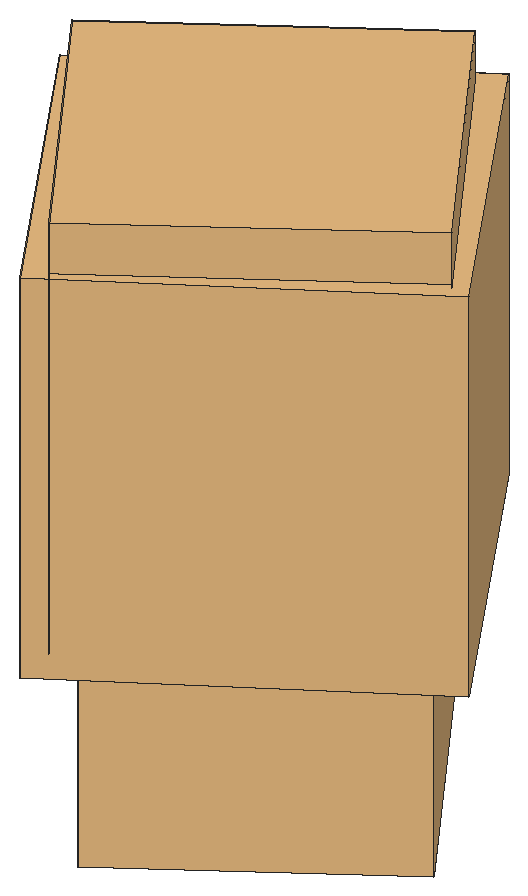
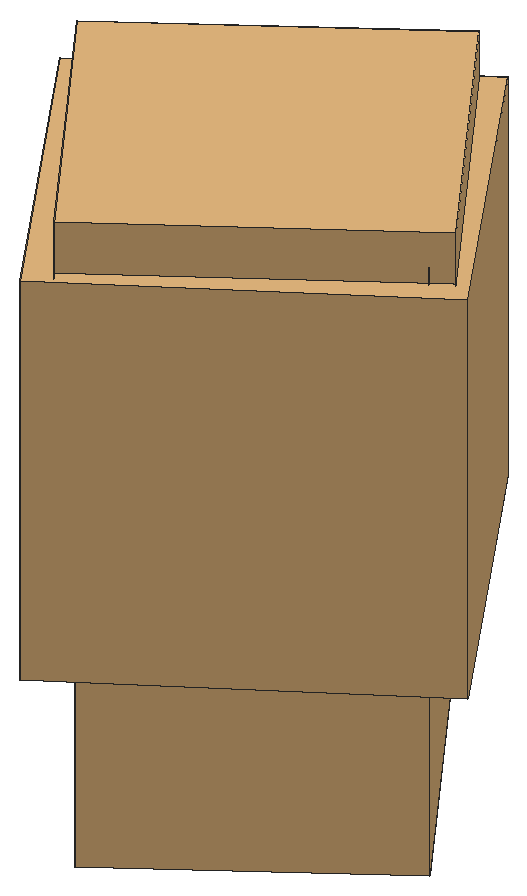
# SketchUp Ruby script. Lengths in inches.
U = 1.inch
M = Sketchup.active_model
def pt(a) = Geom::Point3d.new(a.map { |v| v * U })
def face(e, loops, mat)
  f = e.add_face(loops[0].map { |a| pt(a) })
  loops[1..].each { |l| e.add_face(l.map { |a| pt(a) }).erase! }
  f.material = f.back_material = mat if mat
  f
end
# faces: each face lists its corners as indices into pts; further lists are holes
def faces(e, pts, list, mat = nil) = list.each { |f| face(e, (f[0].is_a?(Array) ? f : [f]).map { |l| l.map { |i| pts[i] } }, mat) }
# xy, xz, yz: faces in a plane at the given z, y or x. An outline is a flat list of corners, or four numbers for a rectangle; further outlines are holes
def ring(l) = l.size == 4 ? [[l[0], l[1]], [l[2], l[1]], [l[2], l[3]], [l[0], l[3]]] : l.each_slice(2).to_a
def flat(e, list, mat, &to3) = list.each { |f| face(e, (f[0].is_a?(Array) ? f : [f]).map { |l| ring(l).map { |u, v| to3.(u, v) } }, mat) }
def xy(e, z, list, mat = nil) = flat(e, list, mat) { |x, y| [x, y, z] }
def xz(e, y, list, mat = nil) = flat(e, list, mat) { |x, z| [x, y, z] }
def yz(e, x, list, mat = nil) = flat(e, list, mat) { |y, z| [x, y, z] }
def lines(e, pts, list) = list.each { |a, b| e.add_line(pt(pts[a]), pt(pts[b])) }
# prism: a flat outline (further loops are holes) pulled along v
def prism(e, loops, v, mat = nil)
  f = face(e, loops, mat); d = Geom::Vector3d.new(v.map { |x| x * U })
  f.pushpull(f.normal.samedirection?(d) ? d.length : -d.length)
end
def box(e, o, s, mat = nil) = prism(e, [[o, [o[0] + s[0], o[1], o[2]], [o[0] + s[0], o[1] + s[1], o[2]], [o[0], o[1] + s[1], o[2]]]], [0, 0, s[2]], mat)
def at(x, y, z, deg = 0) = Geom::Transformation.translation(pt([x, y, z])) * Geom::Transformation.rotation(ORIGIN, Z_AXIS, deg.degrees)
def axes(o, x, y, z) = Geom::Transformation.new([*x, 0, *y, 0, *z, 0, *pt(o).to_a, 1])
def part(name) = M.definitions.add(name)
# library, detail: a bought-in or finely detailed component or shape, given as its bounding box
def library(name, o, s) = part(name).tap { |d| box(d.entities, o, s) }
def detail(e, o, s) = box(e.add_group.entities, o, s)
def put(e, d, t, mat = nil) = e.add_instance(d, t).tap { |i| i.material = mat if mat }
def group(e, t, mat = nil) = e.add_group.tap { |g| g.transformation = t; g.material = mat if mat }.entities
root = M.entities
M.materials.add("028_190k_fullGeometry_Material \#4").color = [120, 148, 64]
M.materials.add("0ad16as01f6asdLeafVar1sfd015as60f1as6").color = [231, 235, 211]
M.materials.add("asdfasdf0165f6asdLeafVar1sfd015as60f1as6").color = [231, 235, 211]
M.materials.add("dw_stemssadfasdfa0sdf1s01d6w1").color = [90, 97, 50]
M.materials.add("viburnumblaasdfas0df1w06d").color = [98, 102, 84]
M.materials.add("viburnumbladsadfasdfad0w122").color = [125, 129, 119]
c1 = part("Component\#314")
p = [[0.14,0,0],[2.58,0.05,0.25],[2.44,5.11,2.64],[0,5.05,2.39]]
faces(c1.entities,p,[[0,1,2,3]],"viburnumblaasdfas0df1w06d")
c2 = part("viburnumblad1\#2")
put(c2.entities,c1,axes([-37.25,6.23,19.31],[75.98784,0,0],[0,65.50676,0],[0,0,75.98784]))
c3 = library("028_190k_fullGeometry_0",[-319.99,-281.1,-2.15],[577.33,562.38,1159.36])
c4 = library("028_190k_fullGeometry_1",[-333.4,-281.7,421.48],[600.33,578.53,738.83])
c5 = library("028_190k_fullGeometry_2",[-3584003,-3264710,4041818.25],[6566285.5,6460741.75,7903602.75])
c6 = library("028_190k_fullGeometry_3",[-353.86,-324.57,405.22],[652.24,636.69,781.83])
c7 = part("028_190k_fullGeometry_4")
p = [[125.51,152.8,882.93],[125.36,152.82,883.01],[124.8,155.5625,881.05]]
faces(c7.entities,p,[[0,1,2]],"028_190k_fullGeometry_Material \#4")
c8 = part("028_190k_fullGeometry")
g1 = group(c8.entities,at(0,0,0))
put(g1,c3,axes([0,0,0],[0.18998,-0.26642,0],[0.26642,0.18998,0],[0,0,0.32722]))
put(g1,c4,axes([0,0,0],[0.18998,-0.26642,0],[0.26642,0.18998,0],[0,0,0.32722]))
put(g1,c5,axes([0,0,0],[0.00002,-0.00003,0],[0.00003,0.00002,0],[0,0,0.00003]))
put(g1,c6,axes([0,0,0],[0.18998,-0.26642,0],[0.26642,0.18998,0],[0,0,0.32722]))
put(g1,c7,axes([0,0,0],[0.18998,-0.26642,0],[0.26642,0.18998,0],[0,0,0.32722]))
c9 = part("Component\#315")
p = [[0.25,0,0],[2.05,0.01,0.35],[1.81,4.2,1.66],[0,4.19,1.3125]]
faces(c9.entities,p,[[0,1,2,3]],"viburnumbladsadfasdfad0w122")
c10 = part("viburnumblad2")
put(c10.entities,c9,axes([-19.23,-4.49,-32.18],[83.35428,0,0],[0,79.38502,0],[0,0,83.35428]))
c11 = part("vdw_leaf\#1")
p = [[0,0,0],[-2.77,1.61,2.32],[-4.3125,6.1,4.5],[-3.97,13.49,6.09],[-2.47,18.57,6.3],[-0.2,22.73,5.75],
  [2.54,19.66,6.85],[4.3,15.93,7.09],[5.03,7.6,5.43],[3.32,1.76,2.74]]
faces(c11.entities,p,[[0,1,2,3,4,5],[0,5,6,7,8,9]],"0ad16as01f6asdLeafVar1sfd015as60f1as6")
c12 = part("dw_branch_3\#2")
p = [[-10.06,-1.6,62.9],[-0.2,1.54,-0.01],[-10.43,1.54,62.72],[0.18,-1.6,0.17],[-23.75,-21.66,88.91],[-25.7,-20.3,89.55],
  [13.4,11.62,104.56],[13.33,13.52,104.47],[-49.25,-41.87,130.3125],[-50.33,-40.21,130.71],[-4.97,21.13,143.98],[35.61,27.99,178.64],
  [-5.09,23.64,143.96],[35.32,29.14,178.46],[-67.7,-55.38,181.06],[-68.34,-54.45,181.62],[-22.8125,33.9,200.59],[-22.94,35.79,200.41],
  [56.61,36.78,229.75],[56.29,38.09,229.57],[-70.63,-67.46,248.85],[-70.72,-66.33,249.5],[-25.05,43.32,240.75],[-24.98,44.26,240.57]]
faces(c12.entities,p,[[0,1,2],[0,3,1],[4,2,5],[4,0,2],[6,0,2],[6,2,7],[8,4,5],[8,5,9],
  [10,6,7],[11,6,7],[10,7,12],[11,7,13],[14,8,9],[14,9,15],[16,10,12],[16,12,17],
  [18,11,13],[18,13,19],[20,14,15],[20,15,21],[22,16,17],[22,17,23]],"dw_stemssadfasdfa0sdf1s01d6w1")
c13 = part("dw_branch3\#2")
put(c13.entities,c11,axes([-70.33,-63.58,233.32],[-1.00752,0.412,0.78596],[-0.24851,-1.22189,0.32195],[0.83141,0.09817,1.01433]))
put(c13.entities,c11,axes([-66.93,-54.91,182.82],[-0.84976,-0.98359,0.33619],[0.99572,-0.74889,0.32577],[-0.05223,0.46521,1.22907]))
put(c13.entities,c11,axes([-46.12,-39.49,126.35],[1.23843,0.5364,0.23552],[-0.56438,0.94474,0.81599],[0.15707,-0.83465,1.07498]))
put(c13.entities,c11,axes([13.0625,13.13,104.77],[-1.01271,0.69982,-0.26884],[-0.74268,-0.99813,0.19939],[-0.10222,0.31872,1.21473]))
put(c13.entities,c11,axes([-18.87,30.42,186.42],[0.36309,1.06515,-0.56675],[-1.14134,0.49515,0.19939],[0.39128,0.45593,1.10754]))
put(c13.entities,c11,axes([-3.2,4.15,75.77],[-1.04153,0.55414,0.44243],[-0.23365,-1.01045,0.71554],[0.6695,0.50943,0.93801]))
put(c13.entities,c11,axes([23.2,19.41,136.3],[-0.65687,-1.11295,-0.05714],[1.05857,-0.61429,-0.20411],[0.15163,-0.1536,1.24868]))
put(c13.entities,c11,axes([-25.57,35.48,201.32],[-0.64726,0.62827,0.87973],[-0.71635,-1.0172,0.19939],[0.80962,-0.39773,0.87973]))
put(c13.entities,c11,axes([-36.37,-32.14,110.35],[-0.80747,1.09962,0.12544],[-0.83333,-0.50188,-0.96467],[-0.72833,-0.64487,0.96467]))
put(c13.entities,c11,axes([-9.89,26.72,156.79],[0.45529,1.02969,0.56572],[-1.16919,0.33753,0.32662],[0.11537,-0.64297,1.07744]))
put(c13.entities,c11,axes([-26.57,46.1,241.0625],[0.00015,0.80921,0.22536],[-0.83985,0.00446,-0.01542],[-0.01605,-0.22532,0.80906]))
put(c13.entities,c11,axes([-9.2,-2.58,61.06],[-1.10001,-0.40312,0.39014],[0.40883,-1.1116,0.00411],[0.35732,0.13566,1.14763]))
put(c13.entities,c11,axes([-69.91,-63.11,233.93],[1.36249,-0.1432,0],[0.13201,1.25603,0.5309],[-0.05549,-0.52799,1.26295]))
put(c13.entities,c11,axes([32.2,25.46,166.13],[0.06878,-1.29051,-0.05714],[1.22165,0.07415,-0.20411],[0.2113,-0.04403,1.24868]))
put(c13.entities,c11,axes([-5.68,-0.66,44.43],[-0.48448,-1.12287,0.17078],[0.98138,-0.33653,0.57135],[-0.48308,0.36756,1.04626]))
put(c13.entities,c11,axes([43.45,32.81,198.64],[0.5408,1.19584,0.14106],[-0.94242,0.32409,0.86557],[0.74952,-0.45533,0.98656]))
put(c13.entities,c11,axes([12.52,14.14,104.98],[1.02694,0.54888,0.41092],[-0.53566,1.05407,-0.06927],[-0.38969,-0.12321,1.13846]))
put(c13.entities,c11,axes([44.55,32.375,198.73],[-0.65687,-1.11295,-0.05714],[1.05857,-0.61429,-0.20411],[0.15163,-0.1536,1.24868]))
put(c13.entities,c11,axes([-5.67,21.17,141.44],[-1.10726,0.43603,-0.32953],[-0.49537,-1.03435,0.29588],[-0.17521,0.40597,1.12589]))
put(c13.entities,c11,axes([55.69,37.84,229.48],[0.18984,0.96334,0.18958],[-0.71996,0.0053,0.69399],[0.66755,-0.26823,0.69457]))
put(c13.entities,c11,axes([-21.52,36.85,205.2],[0.72606,-0.98817,0.14519],[0.94364,0.7084,0.10251],[-0.16885,0.05176,1.19664]))
put(c13.entities,c11,axes([-68.51,-56.35,196.07],[1.16319,0.72381,0],[-0.66725,1.0723,0.5309],[0.28049,-0.45075,1.26295]))
put(c13.entities,c12,at(0.01,-0.09,-0.02),"dw_stemssadfasdfa0sdf1s01d6w1")
put(c13.entities,c11,axes([-2.49,5.18,75.91],[0.78614,-0.90346,-0.30078],[0.86953,0.79562,-0.11715],[0.28546,-0.14014,1.16705]))
put(c13.entities,c11,axes([-23.125,-16.22,82.25],[0.32175,1.32576,0.12544],[-1.33153,0.31835,0.05068],[0.01989,-0.13382,1.3633]))
put(c13.entities,c11,axes([-23.75,41.99,230.3],[0.85958,-0.87451,0.14519],[0.66531,0.75721,0.62192],[-0.54076,-0.36226,1.01955]))
put(c13.entities,c11,axes([27.07,22.48,149.34],[0.92952,-0.64745,-0.62467],[0.50188,1.074,-0.36637],[0.71693,0.02135,1.04468]))
put(c13.entities,c11,axes([17.66,16.25,119.93],[-0.91649,0.83891,-0.3601],[-0.87434,-0.77966,0.40896],[0.0492,0.54447,1.14321]))
put(c13.entities,c11,axes([-68.37,-54.54,181.63],[0.32047,1.28399,0.35434],[-1.33153,0.31835,0.05068],[-0.03484,-0.35624,1.32241]))
put(c13.entities,c11,axes([-28.98,-27.1,96.48],[-0.8814,-0.35966,-0.98523],[0.75246,-1.11336,-0.26672],[-0.73065,-0.71272,0.91382]))
put(c13.entities,c11,axes([-15.23,28.43,172.72],[-1.21149,0.11898,0.32517],[-0.09739,-1.25259,0.09551],[0.33228,0.0667,1.21356]))
put(c13.entities,c11,axes([-17.5625,31.23,186.85],[-0.49275,-1.12287,0.14519],[0.95014,-0.33653,0.62192],[-0.53717,0.36756,1.01955]))
put(c13.entities,c11,axes([26.7,21.22,149.39],[-1.00104,0.22334,0.83093],[0.36894,-1.0402,0.72406],[0.77731,0.78134,0.72643]))
put(c13.entities,c11,axes([-31.125,-24.87,97.38],[0.75482,-0.86936,0.69068],[-0.00159,0.80023,1.00899],[-1.08766,-0.58016,0.45842]))
put(c13.entities,c11,axes([-71.21,-66.73,248.67],[0.25207,0.96771,0],[-0.8921,0.23237,0.38752],[0.375,-0.09768,0.92186]))
put(c13.entities,c11,axes([-24.11,41.05,229.55],[-1.11612,0.51924,-0.26884],[-0.56394,-1.10897,0.19939],[-0.15444,0.29694,1.21473]))
put(c13.entities,c11,axes([6.75,8.37,91.63],[-0.33418,-1.12287,0.39014],[1.13558,-0.33653,0.00411],[0.10478,0.36756,1.14763]))
put(c13.entities,c11,axes([-26,45.89,241.63],[-0.26986,-0.70824,-0.32129],[0.56818,-0.39091,0.38449],[-0.49365,-0.09775,0.63011]))
put(c13.entities,c11,axes([3.74,17.32,124.35],[0.22441,1.22913,-0.16274],[-1.07812,0.11178,-0.64246],[-0.61228,0.25367,1.07162]))
put(c13.entities,c11,axes([-5.44,22.27,140.88],[1.2203,0.00475,0.31374],[-0.097,1.20386,0.35905],[-0.29841,-0.37189,1.1663]))
put(c13.entities,c11,axes([-13.79,29.35,173.31],[0.83169,-0.90108,0.14519],[0.68877,0.73594,0.62192],[-0.55187,-0.34509,1.01955]))
put(c13.entities,c11,axes([-16.92,-7.26,72.98],[1.30647,0.30378,-0.27886],[0.07026,0.74892,1.14503],[0.40633,-1.10623,0.69861]))
put(c13.entities,c11,axes([4.8,17.55,125.22],[-0.25598,-1.17842,0.26559],[1.01553,-0.08455,0.60363],[-0.56975,0.35087,1.00767]))
put(c13.entities,c11,axes([5.3125,8.35,91.45],[0.00638,1.22913,-0.27714],[-1.16413,0.11178,0.46895],[0.48205,0.25367,1.13617]))
put(c13.entities,c11,axes([38.12,30.57,183.07],[1.12534,0.26182,-0.63833],[-0.46674,1.18829,-0.33545],[0.5081,0.51169,1.10563]))
put(c13.entities,c11,axes([-70.41,-60.38,214.47],[-0.41425,1.30587,0],[-1.20383,-0.38188,0.5309],[0.50605,0.16053,1.26295]))
put(c13.entities,c11,axes([37.03,28.75,180.67],[-1.12533,0.00102,-0.63799],[-0.00113,-1.2408,0],[-0.62497,0.00057,1.10237]))
put(c13.entities,c11,axes([30.71,25.35,165.96],[-0.1364,1.29314,0.22715],[-1.08768,-0.23921,0.70862],[0.73536,-0.11394,1.09026]))
put(c13.entities,c11,axes([-38.05,-30.84,110.67],[-0.31533,-1.27379,-0.2839],[1.018,-0.40311,0.67794],[-0.74394,-0.05723,1.08307]))
put(c13.entities,c11,axes([50.11,34.45,213.36],[-1.05669,0.74401,-0.05714],[-0.616,-0.82138,0.69675],[0.37221,0.60904,1.04705]))
put(c13.entities,c11,axes([-65.32,-58.78,200.07],[-1.14597,-0.19668,-0.6713],[0.21784,-1.26924,0],[-0.64812,-0.11124,1.139]))
put(c13.entities,c11,axes([-53.2,-43.37,143.59],[-0.72817,-1.09167,-0.2839],[0.82127,-0.72411,0.67794],[-0.71934,0.19815,1.08307]))
put(c13.entities,c11,axes([-61.1,-50.25,163.67],[-0.52887,1.19686,-0.30066],[-1.10762,-0.57104,-0.32484],[-0.42634,0.12264,1.23812]))
put(c13.entities,c11,axes([-54.12,-42.96,142.67],[0.32175,1.32576,0.12544],[-1.33153,0.31835,0.05068],[0.01989,-0.13382,1.3633]))
put(c13.entities,c11,axes([22.03,20.08,132.3],[1.17066,0.5058,-0.34078],[-0.35758,1.16671,0.50333],[0.49407,-0.35407,1.17172]))
put(c13.entities,c11,axes([-8.59,26.04,158.21],[-0.49275,-1.12287,0.14519],[0.95014,-0.33653,0.62192],[-0.53717,0.36756,1.01955]))
put(c13.entities,c11,axes([49.92,34.03,213.7],[1.24742,-0.35176,0.25024],[0.42127,1.159,-0.4708],[-0.09426,0.52477,1.20753]))
put(c13.entities,c11,axes([-70.34,-67.02,249.05],[-0.57048,-0.79684,0],[0.73827,-0.52855,0.24329],[-0.20203,0.14464,0.92729]))
put(c13.entities,c11,axes([56.04,36.81,228.63],[0.33451,-0.90845,-0.15237],[0.87636,0.33365,-0.06538],[0.11487,-0.11636,0.94597]))
put(c13.entities,c11,axes([-69.93,-60.58,214.88],[-0.45293,-0.99272,-0.78227],[1.14635,-0.58199,0.07483],[-0.40282,-0.65636,1.06615]))
put(c13.entities,c11,axes([-16.77,-8.59,72.7],[-1.22785,0.11509,0.53076],[-0.24879,-1.22495,-0.30991],[0.46742,-0.38989,1.16587]))
put(c13.entities,c11,axes([18.29,17.18,119.24],[1.19981,-0.45946,0.3029],[0.40159,1.22775,0.27158],[-0.37626,-0.1547,1.25575]))
put(c13.entities,c11,axes([-6.73,-0.68,43.74],[0.05346,1.22913,-0.27201],[-1.22696,0.11178,0.26396],[0.28163,0.25367,1.20164]))
put(c13.entities,c11,axes([-58.57,-48.42,160.98],[0.43385,-1.23789,0.39533],[1.04879,0.57965,0.66404],[-0.76727,0.09236,1.13122]))
put(c13.entities,c11,axes([-23.4,38.49,215.38],[0.06762,1.22913,-0.26884],[-1.23909,0.11178,0.19939],[0.21835,0.25367,1.21473]))
put(c13.entities,c11,axes([-22.21,-16.62,83.17],[-0.72817,-1.09167,-0.2839],[0.82127,-0.72411,0.67794],[-0.71934,0.19815,1.08307]))
put(c13.entities,c11,axes([-45.7,-40.77,126.53],[-1.33715,-0.0713,-0.0976],[0.07167,-1.28508,-0.04314],[-0.09306,-0.0492,1.31098]))
put(c13.entities,c11,axes([-22.39,38.51,216.12],[-0.49275,-1.12287,0.14519],[0.95014,-0.33653,0.62192],[-0.53717,0.36756,1.01955]))
c14 = part("vdw_leaf\#2")
p = [[0,0,0],[-2.77,1.61,2.32],[-4.3125,6.1,4.5],[-3.97,13.49,6.09],[-2.47,18.57,6.3],[-0.2,22.73,5.75],
  [2.54,19.66,6.85],[4.3,15.93,7.09],[5.03,7.6,5.43],[3.32,1.76,2.74]]
faces(c14.entities,p,[[0,1,2,3,4,5],[0,5,6,7,8,9]],"asdfasdf0165f6asdLeafVar1sfd015as60f1as6")
c15 = part("dg_branch_1\#2")
p = [[46.12,1.57,35.62],[46,5.42,35.41],[0.14,1.79,0.05],[0.26,-2.0625,0.27],[74.05,2.99,75.8],[74.11,5.28,75.58],
  [103.46,0.47,94.74],[104.03,2.92,94.84],[81.14,16.92,120.46],[81.2,18.78,120.24],[130.47,-5.6875,130.27],[130.58,-3.66,129.85],
  [80.82,34.4375,191.22],[80.64,35.93,190.9],[148.49,-14.56,203.24],[148.9,-12.8125,203.11],[81.08,37.95,226.93],[81.4,39.1,227.03],
  [157.45,-18.19,250.77],[157.7,-17.01,250.41]]
faces(c15.entities,p,[[0,1,2,3],[4,0,1],[4,1,5],[6,4,5],[6,5,7],[8,4,5],[8,5,9],[10,6,7],
  [10,7,11],[12,8,9],[12,9,13],[14,10,11],[14,11,15],[16,12,13],[16,13,17],[18,14,15],
  [18,15,19]],"dw_stemssadfasdfa0sdf1s01d6w1")
c16 = part("vdw_branch1\#3")
put(c16.entities,c14,axes([120.69,-2.42,117.31],[1.12221,-0.24063,-0.65809],[0.19207,1.24776,-0.12871],[0.65778,0.01392,1.11658]))
put(c16.entities,c14,axes([81,38.9,226.05],[0.7888,-0.58155,0],[0.48308,0.65523,0.47],[-0.28484,-0.38635,0.83138]))
put(c16.entities,c14,axes([78.08,12.69,106.05],[-1.43826,-0.02353,-0.03177],[0.0088,-1.31777,0.57755],[-0.03854,0.57714,1.31741]))
put(c16.entities,c14,axes([130.18,-4.73,130.41],[-0.38031,-1.29044,-0.11242],[1.20662,-0.31032,-0.51987],[0.47109,-0.24694,1.24081]))
put(c16.entities,c14,axes([157.08,-17.89,249.93],[-0.91355,0.40674,0],[-0.37496,-0.84216,0.38752],[0.15762,0.35401,0.92186]))
put(c16.entities,c14,axes([90.64,3.03,86.49],[0.32514,-0.85045,-0.99675],[0.69523,0.98247,-0.61148],[1.11061,-0.36604,0.67459]))
put(c16.entities,c14,axes([80.15,28.42,160.95],[-0.16039,0.95636,-1.06292],[-1.41646,0.03966,0.24943],[0.19509,1.07422,0.93709]))
put(c16.entities,c14,axes([126.74,-5.45,129.22],[-0.59819,0.96152,-0.6841],[-0.85772,0.12575,0.92675],[0.75427,0.88089,0.57856]))
put(c16.entities,c14,axes([133.22,-6.12,150.66],[-0.93823,0.76985,0.59124],[-0.47726,-1.08188,0.65135],[0.84525,0.24366,1.02405]))
put(c16.entities,c14,axes([80.43,22.89,141.32],[-1.42571,-0.19312,0.01373],[0.18338,-1.31425,0.5561],[-0.0621,0.5528,1.32692]))
put(c16.entities,c14,axes([33.14,0.88,26.42],[-0.13338,1.31536,0.04876],[-1.04528,-0.13221,0.7073],[0.72315,0.03348,1.07497]))
put(c16.entities,c14,axes([152.63,-15.08,221.76],[-1.28188,0.41945,0.0579],[-0.3638,-1.18547,0.53367],[0.21665,0.49113,1.23869]))
put(c16.entities,c14,axes([80.05,28.28,160.33],[-0.46732,-1.26661,0.40679],[1.27397,-0.40257,0.21004],[-0.07408,0.44645,1.30501]))
put(c16.entities,c14,axes([153.95,-14.8,235.875],[0.39005,1.07743,0.20605],[-0.96443,0.25296,0.50293],[0.42961,-0.3464,0.99807]))
put(c16.entities,c14,axes([80.2,24.22,141.74],[1.33062,-0.46576,0.02628],[0.44746,1.2746,-0.06608],[-0.00197,0.0722,1.37936]))
put(c16.entities,c14,axes([145.48,-12.5,188.92],[-1.32952,0.16983,0.16138],[-0.09299,-1.2361,0.53471],[0.21503,0.51548,1.22904]))
put(c16.entities,c14,axes([139.64,-9.18,171.24],[0.05682,1.30088,0.23414],[-1.13176,-0.05343,0.57151],[0.58357,-0.22963,1.13417]))
put(c16.entities,c14,axes([70.95,4.35,71.98],[-1.1081,-0.41873,0.64752],[0.33675,-1.28259,-0.25313],[0.6937,-0.04625,1.15721]))
put(c16.entities,c14,axes([59.85,4.55,56.17],[-0.26797,1.24526,0.35754],[-0.9369,-0.41634,0.74783],[0.83377,-0.10389,0.98674]))
put(c16.entities,c14,axes([33.11,3.36,25.66],[-0.57817,-1.07968,-0.5679],[1.11554,-0.21356,-0.7297],[0.49375,-0.78178,0.98363]))
put(c16.entities,c15,at(-0.21,0.34,-0.17),"dw_stemssadfasdfa0sdf1s01d6w1")
put(c16.entities,c14,axes([80.91,19.01,122.53],[-0.84258,1.13222,-0.27981],[-1.15093,-0.75138,0.42537],[0.18861,0.47293,1.3457]))
put(c16.entities,c14,axes([119.8,-1.22,114.1],[-1.3235,-0.25012,0.09101],[0.25933,-1.31572,0.15537],[0.05991,0.1698,1.33794]))
put(c16.entities,c14,axes([46.29,5.1,38.04],[0.98937,0.73827,-0.47585],[-0.72359,1.03721,0.10473],[0.44068,0.18581,1.20453]))
put(c16.entities,c14,axes([81.1875,33.03,184.45],[1.33883,0.26986,0.35053],[-0.09581,1.22087,-0.57399],[-0.42216,0.53228,1.20262]))
put(c16.entities,c14,axes([80.16,36.28,206.98],[-0.83993,0.85737,-0.6234],[-1.05964,-0.65701,0.5241],[0.02941,0.81391,1.07976]))
put(c16.entities,c14,axes([154.86,-16.15,234.87],[0.02509,-1.15302,-0.28506],[1.1487,-0.04894,0.29908],[-0.30202,-0.28195,1.11384]))
put(c16.entities,c14,axes([108.77,-0.33,101.14],[-0.47691,-1.03266,-0.72709],[1.25395,-0.29455,-0.40416],[0.15052,-0.81814,1.06325]))
put(c16.entities,c14,axes([89.79,3.01,85.87],[-0.61344,0.75518,0.8965],[-0.17758,-1.01824,0.73622],[1.13385,0.22574,0.58569]))
put(c16.entities,c14,axes([81.56,20.31,123.29],[0.37259,-1.3435,0.21057],[1.29385,0.32364,-0.22445],[0.16906,0.25791,1.34638]))
put(c16.entities,c14,axes([46.45,1.82,36.74],[-0.77883,0.29892,1.0614],[0.19124,-1.24314,0.49044],[1.08598,0.43329,0.67484]))
put(c16.entities,c14,axes([71.37,4.02,72.32],[0.72905,0.81546,-0.74421],[-0.66805,0.98958,0.42988],[0.8391,0.14186,0.97745]))
put(c16.entities,c14,axes([136.59,-5.88,150.53],[0.85845,-0.99897,-0.12437],[0.96526,0.81273,0.13453],[-0.02572,-0.18182,1.28292]))
put(c16.entities,c14,axes([80.375,38.8,225.86],[-0.25178,0.96778,0],[-0.89216,-0.23211,0.38752],[0.37503,0.09757,0.92186]))
put(c16.entities,c14,axes([74.43,7.99,85.38],[-1.05703,0.91669,-0.33543],[-0.95806,-0.87958,0.61531],[0.18697,0.6754,1.25659]))
put(c16.entities,c14,axes([76.57,9.74,89.32],[0.63146,-1.21538,0.33508],[1.18148,0.49387,-0.43517],[0.26321,0.48577,1.26593]))
put(c16.entities,c14,axes([81.6875,36.97,207.4],[0.09422,-1.04424,0.38486],[1.01646,0.1939,0.27727],[-0.33299,0.33382,0.98727]))
put(c16.entities,c14,axes([157.29,-17.17,249.98],[0.50586,-0.50586,0],[0.38853,0.38853,0.41105],[-0.29684,-0.29684,0.56115]))
put(c16.entities,c14,axes([79.92,15.8,106.09],[1.03917,-0.29343,-0.90675],[-0.14587,1.22131,-0.5624],[0.92163,0.5191,0.88824]))
put(c16.entities,c14,axes([61.95,3.88,56.26],[0.41243,-1.28546,0],[1.17466,0.37688,-0.54831],[0.5221,0.16751,1.23363]))
put(c16.entities,c14,axes([151.99,-14.79,208.15],[-0.48571,-1.21723,-0.32393],[1.25386,-0.50033,0],[-0.12005,-0.30087,1.31056]))
put(c16.entities,c14,axes([108.44,0.62,102.22],[0.82183,0.96078,0.38967],[-0.62327,0.08618,1.10203],[0.79141,-0.88661,0.51693]))
put(c16.entities,c14,axes([145.6,-10.56,188.62],[1.03241,-0.02554,-0.82693],[0.3944,1.11584,0.45794],[0.70325,-0.61672,0.89706]))
put(c16.entities,c14,axes([78.59,32.3,183.89],[-1.12675,-0.42036,0.43987],[0.5899,-0.98149,0.57312],[0.14901,0.70693,1.05726]))
put(c16.entities,c14,axes([152.08,-13.42,223.37],[0.79993,-0.44251,-0.69938],[0.68456,0.82615,0.26026],[0.41048,-0.60953,0.85515]))
put(c16.entities,c14,axes([140.71,-8.74,170.55],[0.41903,-1.24177,-0.32393],[1.26224,0.33728,0.33986],[-0.23168,-0.40836,1.26573]))
put(c16.entities,c14,axes([149.25,-12.53,205.78],[1.24456,0.38285,0.23414],[-0.42999,1.04826,0.57151],[-0.02056,-0.62679,1.13417]))
c17 = part("vdw_leaf\#3")
p = [[0,0,0],[-2.77,1.61,2.32],[-4.3125,6.1,4.5],[-3.97,13.49,6.09],[-2.47,18.57,6.3],[-0.2,22.73,5.75],
  [2.54,19.66,6.85],[4.3,15.93,7.09],[5.03,7.6,5.43],[3.32,1.76,2.74]]
faces(c17.entities,p,[[0,1,2,3,4,5],[0,5,6,7,8,9]],"asdfasdf0165f6asdLeafVar1sfd015as60f1as6")
c18 = part("dw_brancj_2\#2")
p = [[9.7,-0.22,29.95],[0.23,-1.96,0.34],[-0.05,1.51,0.11],[9.65,1.51,29.46],[18.64,-8.75,84.43],[18.96,-6.63,84.625],
  [1.53,6.02,63.68],[1.42,8.18,63.25],[-10.58,8.77,161.17],[-10.41,9.98,160.68],[26.34,-9.37,211.72],[26.57,-8.28,211.23]]
faces(c18.entities,p,[[0,1,2],[0,2,3],[4,0,3],[4,3,5],[6,0,3],[6,3,7],[8,6,7],[8,7,9],
  [10,4,5],[10,5,11]],"dw_stemssadfasdfa0sdf1s01d6w1")
c19 = part("vdw_branch2\#3")
put(c19.entities,c17,axes([19.53,-5.9,102.42],[1.12377,-0.50004,0],[0.46097,1.03596,0.47664],[-0.19377,-0.43548,1.13389]))
put(c19.entities,c17,axes([-5.89,6.52,109.44],[-1.07209,0.83679,0],[-0.77141,-0.98832,0.52702],[0.32427,0.41545,1.25373]))
put(c19.entities,c17,axes([-0.44,8.23,75.28],[0.88709,-0.9947,0],[0.92159,0.82189,0.33087],[-0.25219,-0.22491,1.26111]))
put(c19.entities,c17,axes([24.71,-8.97,190.81],[-0.82641,0.91101,0],[-0.83983,-0.76184,0.47664],[0.35303,0.32025,1.13389]))
put(c19.entities,c17,axes([-2.29,8.24,91.35],[1.24603,-0.47303,0],[0.43826,1.15445,0.33087],[-0.11993,-0.31592,1.26111]))
put(c19.entities,c17,axes([12.26,-3.11,37.92],[-0.64625,1.02205,0.22511],[-1.04383,-0.61044,-0.22511],[-0.07533,-0.30931,1.18809]))
put(c19.entities,c17,axes([26.17,-9.17,210.27],[-0.99452,-0.10453,0],[0.09636,-0.91681,0.38752],[-0.04051,0.38539,0.92186]))
put(c19.entities,c17,axes([-6.07,9.4,125.35],[-0.90214,-0.98107,0],[0.90896,-0.83583,0.33087],[-0.24874,0.22873,1.26111]))
put(c19.entities,c17,axes([-4.13,7.29,110.58],[0.44715,-1.078,0.64369],[1.05816,0.63649,0.33087],[-0.58725,0.40856,1.09216]))
put(c19.entities,c17,axes([23.91,-8.22,171.96],[0.62307,0.85009,-0.63406],[-0.71531,0.8798,0.47664],[0.78296,0.12729,0.94004]))
put(c19.entities,c18,at(-0.09,0.18,-0.25),"dw_stemssadfasdfa0sdf1s01d6w1")
put(c19.entities,c17,axes([23.34,-9.65,156.59],[-0.31364,-1.00782,0.58216],[1.10369,-0.17062,0.29925],[-0.17137,0.6239,0.98776]))
put(c19.entities,c17,axes([15.03,-3.37,58.83],[-1.05425,-0.00194,0.58442],[-0.14303,-1.11707,-0.26172],[0.55355,-0.3046,0.99755]))
put(c19.entities,c17,axes([-11.625,9.46,160.37],[0.36812,0.92978,0],[-0.85713,0.33936,0.38752],[0.3603,-0.14265,0.92186]))
put(c19.entities,c17,axes([21.32,-8.53,138.72],[1.21379,0.19904,0],[-0.19904,1.21379,0],[0,0,1.23]))
put(c19.entities,c17,axes([22.54,-9.2,141.43],[-1.02887,0.17955,0.60182],[-0.23387,-1.13057,-0.06253],[0.56696,-0.17376,1.02111]))
put(c19.entities,c17,axes([23.9,-8.82,173.84],[-1.14567,-0.37474,0],[0.35918,-1.0981,0.04438],[-0.01409,0.04308,1.17993]))
put(c19.entities,c17,axes([-7.84,8.92,143.59],[-1.26971,0.40522,0],[-0.37543,-1.17638,0.33087],[0.10274,0.32192,1.26111]))
put(c19.entities,c17,axes([19.77,-8.01,85.98],[-0.32405,-1.14591,0.18674],[1.10278,-0.32969,-0.10948],[0.15845,0.14442,1.16117]))
put(c19.entities,c17,axes([-0.62,5.76,76.34],[-0.08879,1.17576,-0.67771],[-1.34525,-0.16582,-0.11144],[-0.17897,0.66309,1.17383]))
put(c19.entities,c17,axes([20.49,-8.22,121.07],[0.39924,-0.78471,-0.8233],[1.08735,0.33121,0.2116],[0.09035,-0.83005,0.83495]))
put(c19.entities,c17,axes([15.15,-3.72,62.9],[1.16251,0.40128,-0.0211],[-0.39924,1.16074,0.07874],[0.0456,-0.06757,1.2273]))
put(c19.entities,c17,axes([20.72,-8.08,120.26],[-0.03693,1.2277,-0.06551],[-1.22944,-0.03698,0],[-0.00197,0.06548,1.22825]))
put(c19.entities,c17,axes([22.58,-8.36,155.57],[-0.56247,1.09386,0],[-1.00839,-0.51852,0.47664],[0.42389,0.21796,1.13389]))
put(c19.entities,c17,axes([3.97,3.13,57.96],[-1.09459,0.76041,0],[-0.72262,-1.0402,-0.1735],[-0.10109,-0.14552,1.29352]))
put(c19.entities,c17,axes([-10.8,9.06,160.75],[-0.66334,-0.72138,0],[0.66835,-0.61458,0.24329],[-0.1829,0.16818,0.92729]))
put(c19.entities,c17,axes([19.06,-9.3125,103.96],[-1.01345,0.25553,-0.60051],[-0.2265,-1.12952,-0.09839],[-0.59598,0.03076,1.01889]))
put(c19.entities,c17,axes([18.07,-6.2,81.7],[-0.56247,1.09386,0],[-1.00839,-0.51852,0.47664],[0.42389,0.21796,1.13389]))
put(c19.entities,c17,axes([12.95,-0.39,43.31],[0.13044,-1.19832,0],[1.11025,0.12085,0.29925],[-0.30382,-0.03307,1.14057]))
put(c19.entities,c17,axes([2.28,8.28,56.18],[1.32413,-0.31027,0],[0.30923,1.31968,-0.11144],[0.02542,0.1085,1.35543]))
put(c19.entities,c17,axes([-7.55,9.96,143.07],[1.34251,-0.21744,0],[0.20045,1.23761,0.52702],[-0.08426,-0.52024,1.25373]))
put(c19.entities,c17,axes([26.15,-8.25,210.66],[0.94661,-0.25364,0],[0.235,0.87703,0.24329],[-0.06431,-0.24,0.92729]))
put(c19.entities,c17,axes([-6.48,11.37,125.16],[0.64635,1.10315,0.46356],[-1.16569,0.46153,0.52702],[0.27017,-0.6478,1.16488]))
put(c19.entities,c17,axes([25.74,-8.35,191.28],[0.13044,-1.19832,0],[1.11025,0.12085,0.29925],[-0.30382,-0.03307,1.14057]))
put(c19.entities,c17,axes([-5.125,7.47,91.6],[-1.10024,0.63688,0.48318],[-0.78682,-1.00808,-0.46292],[0.14137,-0.65404,1.184]))
put(root,c2,axes([2207.3,352.85,12.18],[0.00521,-0.00318,0.0136],[0.01189,0.01244,-0.00164],[-0.00949,0.00985,0.00593]))
put(root,c2,axes([2207.27,355.04,26.82],[-0.00128,0.01292,-0.00526],[-0.01614,-0.0018,-0.00049],[-0.00098,0.00473,0.0118]))
put(root,c2,axes([2207.25,353.11,18.27],[0.01313,-0.00582,0.00636],[0.00841,0.01593,-0.00278],[-0.00467,0.00494,0.01417]))
put(root,c8,at(2234.3125,348.77,-5.3))
put(root,c10,axes([2219.75,355.04,27.57],[0.00677,-0.00276,-0.00724],[0.0003,0.00981,-0.00339],[0.00756,0.00183,0.00557]))
put(root,c10,axes([2207.21,356,24.83],[0.00715,-0.01146,0.00475],[0.01219,0.00751,-0.00024],[-0.0023,0.00416,0.01351]))
put(root,c2,axes([2205.48,353.52,14.54],[0.01075,0.00741,0.00439],[-0.00265,0.0107,-0.01157],[-0.00831,0.00706,0.00843]))
put(root,c10,axes([2206.73,354.5,23.4],[0.01381,-0.0032,0.00202],[0.00375,0.01421,-0.00318],[-0.00124,0.00342,0.01385]))
put(root,c10,axes([2214.66,355.12,28.47],[0.00829,0.00118,-0.00446],[-0.00277,0.00969,-0.0025],[0.00431,0.00339,0.00782]))
put(root,c10,axes([2214.99,355.33,17.4375],[0.00948,-0.00167,-0.00544],[-0.00216,0.00929,-0.00661],[0.00531,0.00641,0.00728]))
put(root,c10,axes([2206.46,354.45,25.375],[0.01238,0.00695,-0.00189],[-0.0072,0.01199,-0.00308],[0.00008,0.00361,0.01386]))
put(root,c13,axes([2238.99,356.45,10.58],[0.09481,-0.08589,0.04174],[0.08433,0.10034,0.02262],[-0.03765,0.00844,0.15579]))
put(root,c16,axes([2242.62,351.42,7.18],[0.11749,0.04939,0],[-0.04939,0.11749,0],[0,0,0.15683]))
put(root,c10,axes([2215.08,356.28,29],[0.00889,-0.00537,-0.00033],[0.00481,0.00824,-0.00432],[0.00239,0.00342,0.00851]))
put(root,c10,axes([2215.67,356.82,17.63],[0.0086,-0.00684,0.0012],[0.00538,0.00535,-0.00804],[0.0044,0.00684,0.00749]))
put(root,c10,axes([2215.8,355.86,18.64],[0.0048,0.00448,-0.0089],[-0.00793,0.0077,-0.0004],[0.00603,0.00655,0.00655]))
put(root,c2,axes([2207.03,355.61,26.75],[0.00337,0.00858,-0.01052],[-0.01574,0.00327,-0.00237],[0.0008,0.00999,0.00793]))
put(root,c16,axes([2236.12,352.49,7.1875],[-0.11174,0.0797,0],[-0.0797,-0.11174,0],[0,0,0.16889]))
put(root,c2,axes([2208.38,357.92,27.26],[-0.00982,0.00575,-0.00616],[-0.00925,-0.00382,0.01097],[0.00277,0.01054,0.00496]))
put(root,c2,axes([2211.3125,358.33,22.77],[0.0041,-0.00986,0.01208],[0.01717,-0.00172,-0.00723],[0.00492,0.01267,0.00868]))
put(root,c10,axes([2204.05,358.21,17.3125],[0.00529,-0.00535,0.00878],[0.00925,0.00849,-0.00041],[-0.00626,0.00721,0.00817]))
put(root,c10,axes([2215.24,361.1,27.28],[-0.0106,-0.00225,0.00809],[0.00771,-0.01018,0.00728],[0.00487,0.01032,0.00927]))
put(root,c10,axes([2204.25,359.54,18.33],[-0.00352,-0.00882,0.00823],[0.00998,0.00284,0.00731],[-0.00692,0.00849,0.00615]))
put(root,c19,axes([2243.94,350.68,5.57],[0.02729,0.1244,-0.09048],[-0.14364,0.03151,0],[0.01575,0.07182,0.15671]))
put(root,c2,axes([2208.45,360.24,26.95],[-0.01249,0.00074,0.00321],[0.00342,-0.00484,0.01344],[0.00175,0.01171,0.00271]))
put(root,c10,axes([2202.79,360.3,19.07],[0.00504,-0.005,0.01036],[0.00925,0.00849,-0.00041],[-0.00684,0.0078,0.00709]))
